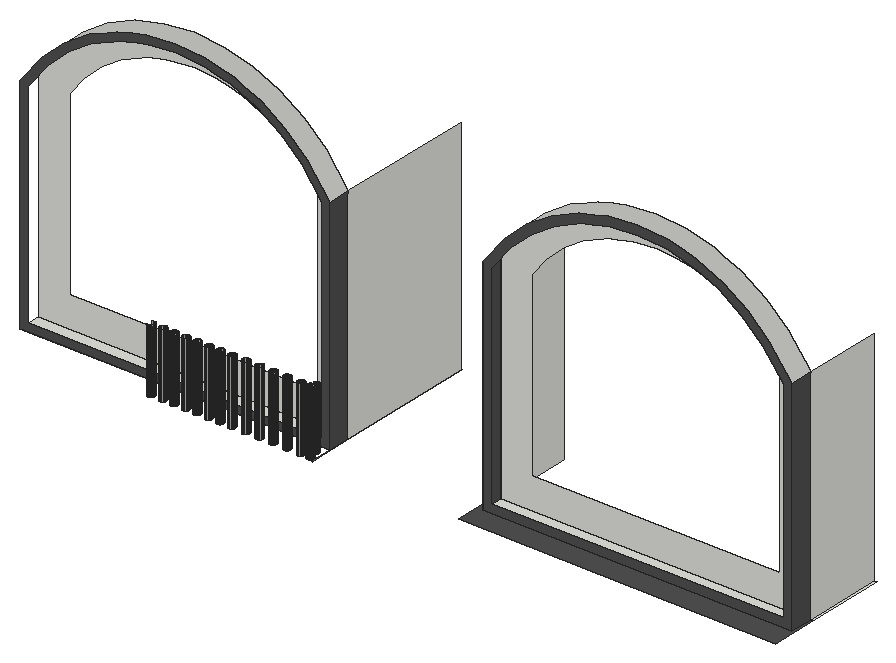
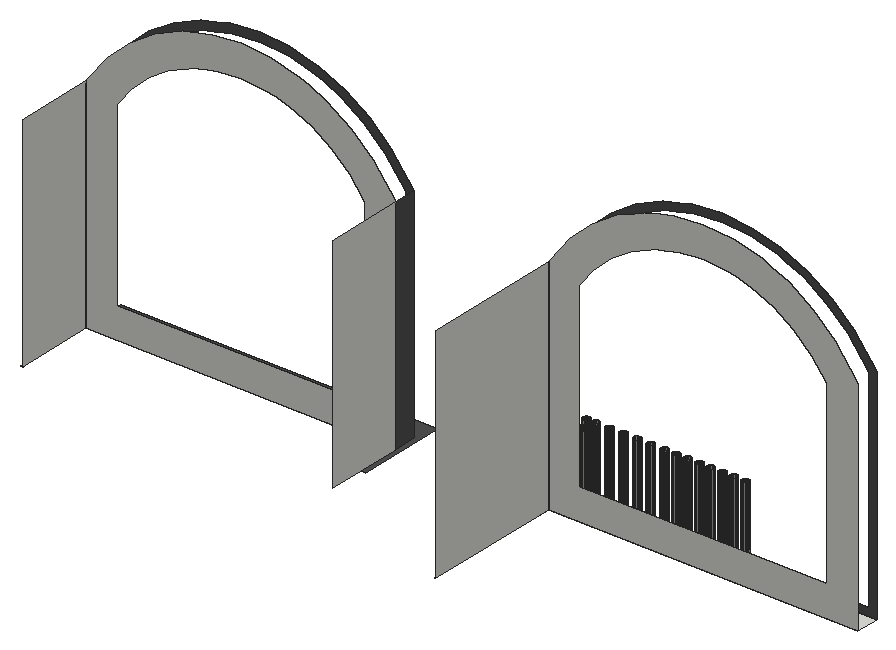
# SketchUp Ruby script. Lengths in inches.
U = 1.inch
M = Sketchup.active_model
def pt(a) = Geom::Point3d.new(a.map { |v| v * U })
def face(e, loops, mat)
  f = e.add_face(loops[0].map { |a| pt(a) })
  loops[1..].each { |l| e.add_face(l.map { |a| pt(a) }).erase! }
  f.material = f.back_material = mat if mat
  f
end
# faces: each face lists its corners as indices into pts; further lists are holes
def faces(e, pts, list, mat = nil) = list.each { |f| face(e, (f[0].is_a?(Array) ? f : [f]).map { |l| l.map { |i| pts[i] } }, mat) }
# xy, xz, yz: faces in a plane at the given z, y or x. An outline is a flat list of corners, or four numbers for a rectangle; further outlines are holes
def ring(l) = l.size == 4 ? [[l[0], l[1]], [l[2], l[1]], [l[2], l[3]], [l[0], l[3]]] : l.each_slice(2).to_a
def flat(e, list, mat, &to3) = list.each { |f| face(e, (f[0].is_a?(Array) ? f : [f]).map { |l| ring(l).map { |u, v| to3.(u, v) } }, mat) }
def xy(e, z, list, mat = nil) = flat(e, list, mat) { |x, y| [x, y, z] }
def xz(e, y, list, mat = nil) = flat(e, list, mat) { |x, z| [x, y, z] }
def yz(e, x, list, mat = nil) = flat(e, list, mat) { |y, z| [x, y, z] }
def lines(e, pts, list) = list.each { |a, b| e.add_line(pt(pts[a]), pt(pts[b])) }
# prism: a flat outline (further loops are holes) pulled along v
def prism(e, loops, v, mat = nil)
  f = face(e, loops, mat); d = Geom::Vector3d.new(v.map { |x| x * U })
  f.pushpull(f.normal.samedirection?(d) ? d.length : -d.length)
end
def box(e, o, s, mat = nil) = prism(e, [[o, [o[0] + s[0], o[1], o[2]], [o[0] + s[0], o[1] + s[1], o[2]], [o[0], o[1] + s[1], o[2]]]], [0, 0, s[2]], mat)
def at(x, y, z, deg = 0) = Geom::Transformation.translation(pt([x, y, z])) * Geom::Transformation.rotation(ORIGIN, Z_AXIS, deg.degrees)
def axes(o, x, y, z) = Geom::Transformation.new([*x, 0, *y, 0, *z, 0, *pt(o).to_a, 1])
def part(name) = M.definitions.add(name)
# library, detail: a bought-in or finely detailed component or shape, given as its bounding box
def library(name, o, s) = part(name).tap { |d| box(d.entities, o, s) }
def detail(e, o, s) = box(e.add_group.entities, o, s)
def put(e, d, t, mat = nil) = e.add_instance(d, t).tap { |i| i.material = mat if mat }
def group(e, t, mat = nil) = e.add_group.tap { |g| g.transformation = t; g.material = mat if mat }.entities
root = M.entities
M.materials.add("[0132_LightGray]").color = [169, 169, 169]
M.materials.add("[0135_DarkGray]").color = [81, 81, 81]
xy(root,638.72,[[299.83,31.93,299.47,31.97,299.14,32.11,298.86,32.33,298.64,32.62,298.5,32.95,298.45,33.3,298.5,33.66,298.64,33.99,298.86,34.28,299.14,34.49,299.47,34.63,299.83,34.68,300.18,34.63,300.52,34.49,300.8,34.28,301.02,33.99,301.16,33.66,301.2,33.3,301.16,32.95,301.02,32.62,300.8,32.33,300.52,32.11,300.18,31.97],[304.33,31.93,303.97,31.97,303.64,32.11,303.36,32.33,303.14,32.62,303,32.95,302.95,33.3,303,33.66,303.14,33.99,303.36,34.28,303.64,34.49,303.97,34.63,304.33,34.68,304.68,34.63,305.02,34.49,305.3,34.28,305.52,33.99,305.66,33.66,305.7,33.3,305.66,32.95,305.52,32.62,305.3,32.33,305.02,32.11,304.68,31.97],[308.83,31.93,308.47,31.97,308.14,32.11,307.86,32.33,307.64,32.62,307.5,32.95,307.45,33.3,307.5,33.66,307.64,33.99,307.86,34.28,308.14,34.49,308.47,34.63,308.83,34.68,309.18,34.63,309.52,34.49,309.8,34.28,310.02,33.99,310.16,33.66,310.2,33.3,310.16,32.95,310.02,32.62,309.8,32.33,309.52,32.11,309.18,31.97],[313.33,31.93,312.97,31.97,312.64,32.11,312.36,32.33,312.14,32.62,312,32.95,311.95,33.3,312,33.66,312.14,33.99,312.36,34.28,312.64,34.49,312.97,34.63,313.33,34.68,313.68,34.63,314.02,34.49,314.3,34.28,314.52,33.99,314.66,33.66,314.7,33.3,314.66,32.95,314.52,32.62,314.3,32.33,314.02,32.11,313.68,31.97],[317.83,31.93,317.47,31.97,317.14,32.11,316.86,32.33,316.64,32.62,316.5,32.95,316.45,33.3,316.5,33.66,316.64,33.99,316.86,34.28,317.14,34.49,317.47,34.63,317.83,34.68,318.18,34.63,318.52,34.49,318.8,34.28,319.02,33.99,319.16,33.66,319.2,33.3,319.16,32.95,319.02,32.62,318.8,32.33,318.52,32.11,318.18,31.97],
  [322.33,31.93,321.97,31.97,321.64,32.11,321.36,32.33,321.14,32.62,321,32.95,320.95,33.3,321,33.66,321.14,33.99,321.36,34.28,321.64,34.49,321.97,34.63,322.33,34.68,322.68,34.63,323.02,34.49,323.3,34.28,323.52,33.99,323.66,33.66,323.7,33.3,323.66,32.95,323.52,32.62,323.3,32.33,323.02,32.11,322.68,31.97],[326.83,31.93,326.47,31.97,326.14,32.11,325.86,32.33,325.64,32.62,325.5,32.95,325.45,33.3,325.5,33.66,325.64,33.99,325.86,34.28,326.14,34.49,326.47,34.63,326.83,34.68,327.18,34.63,327.52,34.49,327.8,34.28,328.02,33.99,328.16,33.66,328.2,33.3,328.16,32.95,328.02,32.62,327.8,32.33,327.52,32.11,327.18,31.97],[331.33,31.93,330.97,31.97,330.64,32.11,330.36,32.33,330.14,32.62,330,32.95,329.95,33.3,330,33.66,330.14,33.99,330.36,34.28,330.64,34.49,330.97,34.63,331.33,34.68,331.68,34.63,332.02,34.49,332.3,34.28,332.52,33.99,332.66,33.66,332.7,33.3,332.66,32.95,332.52,32.62,332.3,32.33,332.02,32.11,331.68,31.97],[336.7,31.93,336.35,31.97,336.02,32.11,335.73,32.33,335.51,32.62,335.375,32.95,335.33,33.3,335.375,33.66,335.51,33.99,335.73,34.28,336.02,34.49,336.35,34.63,336.7,34.68,337.06,34.63,337.39,34.49,337.68,34.28,337.89,33.99,338.03,33.66,338.08,33.3,338.03,32.95,337.89,32.62,337.68,32.33,337.39,32.11,337.06,31.97],[342.08,31.93,341.72,31.97,341.39,32.11,341.11,32.33,340.89,32.62,340.75,32.95,340.7,33.3,340.75,33.66,340.89,33.99,341.11,34.28,341.39,34.49,341.72,34.63,342.08,34.68,342.43,34.63,342.77,34.49,343.05,34.28,343.27,33.99,343.41,33.66,343.45,33.3,343.41,32.95,343.27,32.62,343.05,32.33,342.77,32.11,342.43,31.97],
  [347.45,31.93,347.1,31.97,346.77,32.11,346.48,32.33,346.26,32.62,346.125,32.95,346.08,33.3,346.125,33.66,346.26,33.99,346.48,34.28,346.77,34.49,347.1,34.63,347.45,34.68,347.81,34.63,348.14,34.49,348.43,34.28,348.64,33.99,348.78,33.66,348.83,33.3,348.78,32.95,348.64,32.62,348.43,32.33,348.14,32.11,347.81,31.97],[352.83,31.93,352.47,31.97,352.14,32.11,351.86,32.33,351.64,32.62,351.5,32.95,351.45,33.3,351.5,33.66,351.64,33.99,351.86,34.28,352.14,34.49,352.47,34.63,352.83,34.68,353.18,34.63,353.52,34.49,353.8,34.28,354.02,33.99,354.16,33.66,354.2,33.3,354.16,32.95,354.02,32.62,353.8,32.33,353.52,32.11,353.18,31.97],[358.2,31.93,357.85,31.97,357.52,32.11,357.23,32.33,357.01,32.62,356.875,32.95,356.83,33.3,356.875,33.66,357.01,33.99,357.23,34.28,357.52,34.49,357.85,34.63,358.2,34.68,358.56,34.63,358.89,34.49,359.18,34.28,359.39,33.99,359.53,33.66,359.58,33.3,359.53,32.95,359.39,32.62,359.18,32.33,358.89,32.11,358.56,31.97],[361.31,35.875,361.05,35.93,360.82,36.05,360.62,36.22,360.48,36.4375,360.4,36.6875,360.38,36.95,360.4375,37.2,360.55,37.4375,360.73,37.63,360.95,37.77,361.19,37.85,361.46,37.87,361.71,37.82,361.94,37.7,362.14,37.52,362.28,37.31,362.36,37.06,362.38,36.8,362.32,36.54,362.21,36.31,362.03,36.11,361.8125,35.97,361.57,35.89],[242.82,40.6875,363.51,49.6875],
  [423.07,40.6875,543.76,49.6875],[363.51,49.6875,363.89,104.375],[543.76,49.6875,543.95,80.4375],[543.95,49.6875,544.82,80.4375]])
xy(root,638.72,[[363.51,31.6875,363.89,37.6875],[421.14,31.6875,544.82,31.6875,544.82,49.6875,543.76,49.6875,543.76,40.6875,423.07,40.6875,423.07,66.75,421.14,66.75],[363.51,37.6875,363.89,49.6875]],"[0135_DarkGray]")
xz(root,40.6875,[[[242.82,638.72,363.51,638.72,363.51,725.13,354.58,736.74,346.11,744.61,336.46,750.96,329.5,754.04,325.89,755.63,320.02,757.13,314.6875,758.49,303.17,759.45,291.65,758.49,286.31,757.13,280.45,755.63,276.84,754.04,269.87,750.96,260.22,744.61,251.75,736.74,242.82,725.13],[245.76,641.66,245.76,724.14,253.93,734.75,262.04,742.29,271.28,748.38,278.02,751.35,281.41,752.85,287.03,754.28,292.13,755.58,303.17,756.5,314.2,755.58,319.3,754.28,324.92,752.85,328.3125,751.35,335.05,748.38,344.3,742.29,352.41,734.75,360.57,724.14,360.57,641.66]],[[423.07,638.72,543.76,638.72,543.76,725.13,534.83,736.74,526.36,744.61,516.71,750.96,509.75,754.04,506.14,755.63,500.27,757.13,494.9375,758.49,483.42,759.45,471.9,758.49,466.56,757.13,460.7,755.63,457.09,754.04,450.12,750.96,440.47,744.61,432,736.74,423.07,725.13],[426.42,642.07,426.42,724,434.48,734.47,442.54,741.96,451.73,748.01,458.4375,750.98,461.79,752.46,467.39,753.88,472.45,755.17,483.42,756.09,494.38,755.17,499.45,753.88,505.04,752.46,508.39,750.98,515.1,748.01,524.29,741.96,532.35,734.47,540.41,724,540.41,642.07]]],"[0135_DarkGray]")
xz(root,49.6875,[[[242.82,638.72,242.82,725.13,251.75,736.74,260.22,744.61,269.87,750.96,276.84,754.04,280.45,755.63,286.31,757.13,291.65,758.49,303.17,759.45,314.6875,758.49,320.02,757.13,325.89,755.63,329.5,754.04,336.46,750.96,346.11,744.61,354.58,736.74,363.51,725.13,363.51,638.72],[254.82,650.72,351.51,650.72,351.51,721.05,345.68,728.63,338.68,735.13,330.7,740.39,324.65,743.0625,321.95,744.25,317.06,745.5,312.69,746.61,311.64,746.7,305.64,747.2,303.17,747.41,293.64,746.61,289.27,745.5,284.38,744.25,281.68,743.0625,275.64,740.39,267.65,735.13,260.65,728.63,254.82,721.05]],[[423.07,638.72,423.07,725.13,432,736.74,440.47,744.61,450.12,750.96,457.09,754.04,460.7,755.63,466.56,757.13,471.9,758.49,483.42,759.45,494.9375,758.49,500.27,757.13,506.14,755.63,509.75,754.04,516.71,750.96,526.36,744.61,534.83,736.74,543.76,725.13,543.76,638.72],[435.07,650.72,531.76,650.72,531.76,721.05,525.93,728.63,518.93,735.13,510.95,740.39,504.9,743.0625,502.2,744.25,497.31,745.5,492.94,746.61,483.7,747.38,483.42,747.41,473.89,746.61,469.52,745.5,464.63,744.25,461.93,743.0625,455.89,740.39,447.9,735.13,440.9,728.63,435.07,721.05]]])
yz(root,363.51,[[49.6875,638.72,104.375,725.13]])
yz(root,363.51,[[40.6875,638.72,49.6875,725.13]],"[0135_DarkGray]")
yz(root,423.07,[[49.6875,638.72,80.4375,725.13]])
yz(root,423.07,[[40.6875,638.72,49.6875,725.13]],"[0135_DarkGray]")
yz(root,543.76,[[49.6875,638.72,80.4375,725.13]])
yz(root,543.76,[[40.6875,638.72,49.6875,725.13]],"[0135_DarkGray]")
p = [[299.47,31.97,638.72],[299.83,31.93,638.72],[299.83,31.93,663.85],[299.47,31.97,663.85],[300.18,31.97,638.72],[300.18,31.97,663.85],
  [303.97,31.97,638.72],[304.33,31.93,638.72],[304.33,31.93,663.85],[303.97,31.97,663.85],[304.68,31.97,638.72],[304.68,31.97,663.85],
  [308.47,31.97,638.72],[308.83,31.93,638.72],[308.83,31.93,663.85],[308.47,31.97,663.85],[309.18,31.97,638.72],[309.18,31.97,663.85],
  [312.97,31.97,638.72],[313.33,31.93,638.72],[313.33,31.93,663.85],[312.97,31.97,663.85],[313.68,31.97,638.72],[313.68,31.97,663.85],
  [317.47,31.97,638.72],[317.83,31.93,638.72],[317.83,31.93,663.85],[317.47,31.97,663.85],[318.18,31.97,638.72],[318.18,31.97,663.85],
  [321.97,31.97,638.72],[322.33,31.93,638.72],[322.33,31.93,663.85],[321.97,31.97,663.85],[322.68,31.97,638.72],[322.68,31.97,663.85],
  [326.47,31.97,638.72],[326.83,31.93,638.72],[326.83,31.93,663.85],[326.47,31.97,663.85],[327.18,31.97,638.72],[327.18,31.97,663.85],
  [330.97,31.97,638.72],[331.33,31.93,638.72],[331.33,31.93,663.85],[330.97,31.97,663.85],[331.68,31.97,638.72],[331.68,31.97,663.85],
  [336.35,31.97,638.72],[336.7,31.93,638.72],[336.7,31.93,663.85],[336.35,31.97,663.85],[337.06,31.97,638.72],[337.06,31.97,663.85],
  [341.72,31.97,638.72],[342.08,31.93,638.72],[342.08,31.93,663.85],[341.72,31.97,663.85],[342.43,31.97,638.72],[342.43,31.97,663.85],
  [347.1,31.97,638.72],[347.45,31.93,638.72],[347.45,31.93,663.85],[347.1,31.97,663.85],[347.81,31.97,638.72],[347.81,31.97,663.85],
  [352.47,31.97,638.72],[352.83,31.93,638.72],[352.83,31.93,663.85],[352.47,31.97,663.85],[353.18,31.97,638.72],[353.18,31.97,663.85],
  [357.85,31.97,638.72],[358.2,31.93,638.72],[358.2,31.93,663.85],[357.85,31.97,663.85],[358.56,31.97,638.72],[358.56,31.97,663.85],
  [361.53,31.97,638.72],[361.89,31.93,638.72],[361.89,31.93,663.85],[361.53,31.97,663.85],[362.25,31.97,638.72],[362.25,31.97,663.85],
  [299.14,32.11,638.72],[299.14,32.11,663.85],[300.52,32.11,638.72],[300.52,32.11,663.85],[303.64,32.11,638.72],[303.64,32.11,663.85],
  [305.02,32.11,638.72],[305.02,32.11,663.85],[308.14,32.11,638.72],[308.14,32.11,663.85],[309.52,32.11,638.72],[309.52,32.11,663.85],
  [312.64,32.11,638.72],[312.64,32.11,663.85],[314.02,32.11,638.72],[314.02,32.11,663.85],[317.14,32.11,638.72],[317.14,32.11,663.85],
  [318.52,32.11,638.72],[318.52,32.11,663.85],[321.64,32.11,638.72],[321.64,32.11,663.85],[323.02,32.11,638.72],[323.02,32.11,663.85],
  [326.14,32.11,638.72],[326.14,32.11,663.85],[327.52,32.11,638.72],[327.52,32.11,663.85],[330.64,32.11,638.72],[330.64,32.11,663.85],
  [332.02,32.11,638.72],[332.02,32.11,663.85],[336.02,32.11,638.72],[336.02,32.11,663.85],[337.39,32.11,638.72],[337.39,32.11,663.85],
  [341.39,32.11,638.72],[341.39,32.11,663.85],[342.77,32.11,638.72],[342.77,32.11,663.85],[346.77,32.11,638.72],[346.77,32.11,663.85],
  [348.14,32.11,638.72],[348.14,32.11,663.85],[352.14,32.11,638.72],[352.14,32.11,663.85],[353.52,32.11,638.72],[353.52,32.11,663.85],
  [357.52,32.11,638.72],[357.52,32.11,663.85],[358.89,32.11,638.72],[358.89,32.11,663.85],[361.2,32.11,638.72],[361.2,32.11,663.85],
  [362.58,32.11,638.72],[362.58,32.11,663.85],[300.8,32.33,638.72],[300.8,32.33,663.85],[303.36,32.33,638.72],[303.36,32.33,663.85],
  [305.3,32.33,638.72],[305.3,32.33,663.85],[307.86,32.33,638.72],[307.86,32.33,663.85],[309.8,32.33,638.72],[309.8,32.33,663.85],
  [312.36,32.33,638.72],[312.36,32.33,663.85],[314.3,32.33,638.72],[314.3,32.33,663.85],[316.86,32.33,638.72],[316.86,32.33,663.85],
  [318.8,32.33,638.72],[318.8,32.33,663.85],[321.36,32.33,638.72],[321.36,32.33,663.85],[323.3,32.33,638.72],[323.3,32.33,663.85],
  [325.86,32.33,638.72],[325.86,32.33,663.85],[327.8,32.33,638.72],[327.8,32.33,663.85],[330.36,32.33,638.72],[330.36,32.33,663.85],
  [332.3,32.33,638.72],[332.3,32.33,663.85],[335.73,32.33,638.72],[335.73,32.33,663.85],[337.68,32.33,638.72],[337.68,32.33,663.85],
  [341.11,32.33,638.72],[341.11,32.33,663.85],[343.05,32.33,638.72],[343.05,32.33,663.85],[346.48,32.33,638.72],[346.48,32.33,663.85],
  [348.43,32.33,638.72],[348.43,32.33,663.85],[351.86,32.33,638.72],[351.86,32.33,663.85],[353.8,32.33,638.72],[353.8,32.33,663.85],
  [357.23,32.33,638.72],[357.23,32.33,663.85],[359.18,32.33,638.72],[359.18,32.33,663.85],[360.92,32.33,638.72],[360.92,32.33,663.85],
  [362.86,32.33,638.72],[362.86,32.33,663.85],[301.02,32.62,638.72],[301.02,32.62,663.85],[303.14,32.62,638.72],[303.14,32.62,663.85],
  [305.52,32.62,638.72],[305.52,32.62,663.85],[307.64,32.62,638.72],[307.64,32.62,663.85],[310.02,32.62,638.72],[310.02,32.62,663.85],
  [312.14,32.62,638.72],[312.14,32.62,663.85],[314.52,32.62,638.72],[314.52,32.62,663.85],[316.64,32.62,638.72],[316.64,32.62,663.85],
  [319.02,32.62,638.72],[319.02,32.62,663.85],[321.14,32.62,638.72],[321.14,32.62,663.85],[323.52,32.62,638.72],[323.52,32.62,663.85],
  [325.64,32.62,638.72],[325.64,32.62,663.85],[328.02,32.62,638.72],[328.02,32.62,663.85],[330.14,32.62,638.72],[330.14,32.62,663.85],
  [332.52,32.62,638.72],[332.52,32.62,663.85],[335.51,32.62,638.72],[335.51,32.62,663.85],[337.89,32.62,638.72],[337.89,32.62,663.85],
  [340.89,32.62,638.72],[340.89,32.62,663.85],[343.27,32.62,638.72],[343.27,32.62,663.85],[346.26,32.62,638.72],[346.26,32.62,663.85],
  [348.64,32.62,638.72],[348.64,32.62,663.85],[351.64,32.62,638.72],[351.64,32.62,663.85],[354.02,32.62,638.72],[354.02,32.62,663.85],
  [357.01,32.62,638.72],[357.01,32.62,663.85],[359.39,32.62,638.72],[359.39,32.62,663.85],[360.7,32.62,638.72],[360.7,32.62,663.85],
  [363.08,32.62,638.72],[363.08,32.62,663.85],[301.16,32.95,638.72],[301.16,32.95,663.85],[303,32.95,638.72],[303,32.95,663.85],
  [305.66,32.95,638.72],[305.66,32.95,663.85],[307.5,32.95,638.72],[307.5,32.95,663.85],[310.16,32.95,638.72],[310.16,32.95,663.85],
  [312,32.95,638.72],[312,32.95,663.85],[314.66,32.95,638.72],[314.66,32.95,663.85],[316.5,32.95,638.72],[316.5,32.95,663.85],
  [319.16,32.95,638.72],[319.16,32.95,663.85],[321,32.95,638.72],[321,32.95,663.85],[323.66,32.95,638.72],[323.66,32.95,663.85],
  [325.5,32.95,638.72],[325.5,32.95,663.85],[328.16,32.95,638.72],[328.16,32.95,663.85],[330,32.95,638.72],[330,32.95,663.85],
  [332.66,32.95,638.72],[332.66,32.95,663.85],[335.375,32.95,638.72],[335.375,32.95,663.85],[338.03,32.95,638.72],[338.03,32.95,663.85],
  [340.75,32.95,638.72],[340.75,32.95,663.85],[343.41,32.95,638.72],[343.41,32.95,663.85],[346.125,32.95,638.72],[346.125,32.95,663.85],
  [348.78,32.95,638.72],[348.78,32.95,663.85],[351.5,32.95,638.72],[351.5,32.95,663.85],[354.16,32.95,638.72],[354.16,32.95,663.85],
  [356.875,32.95,638.72],[356.875,32.95,663.85],[359.53,32.95,638.72],[359.53,32.95,663.85],[360.5625,32.95,638.72],[360.5625,32.95,663.85],
  [363.22,32.95,638.72],[363.22,32.95,663.85],[301.2,33.3,638.72],[301.2,33.3,663.85],[302.95,33.3,638.72],[302.95,33.3,663.85],
  [305.7,33.3,638.72],[305.7,33.3,663.85],[307.45,33.3,638.72],[307.45,33.3,663.85],[310.2,33.3,638.72],[310.2,33.3,663.85],
  [311.95,33.3,638.72],[311.95,33.3,663.85],[314.7,33.3,638.72],[314.7,33.3,663.85],[316.45,33.3,638.72],[316.45,33.3,663.85],
  [319.2,33.3,638.72],[319.2,33.3,663.85],[320.95,33.3,638.72],[320.95,33.3,663.85],[323.7,33.3,638.72],[323.7,33.3,663.85],
  [325.45,33.3,638.72],[325.45,33.3,663.85],[328.2,33.3,638.72],[328.2,33.3,663.85],[329.95,33.3,638.72],[329.95,33.3,663.85],
  [332.7,33.3,638.72],[332.7,33.3,663.85],[335.33,33.3,638.72],[335.33,33.3,663.85],[338.08,33.3,638.72],[338.08,33.3,663.85],
  [340.7,33.3,638.72],[340.7,33.3,663.85],[343.45,33.3,638.72],[343.45,33.3,663.85],[346.08,33.3,638.72],[346.08,33.3,663.85],
  [348.83,33.3,638.72],[348.83,33.3,663.85],[351.45,33.3,638.72],[351.45,33.3,663.85],[354.2,33.3,638.72],[354.2,33.3,663.85],
  [356.83,33.3,638.72],[356.83,33.3,663.85],[359.58,33.3,638.72],[359.58,33.3,663.85],[360.52,33.3,638.72],[360.52,33.3,663.85],
  [363.27,33.3,638.72],[363.27,33.3,663.85],[301.16,33.66,638.72],[301.16,33.66,663.85],[303,33.66,638.72],[303,33.66,663.85],
  [305.66,33.66,638.72],[305.66,33.66,663.85],[307.5,33.66,638.72],[307.5,33.66,663.85],[310.16,33.66,638.72],[310.16,33.66,663.85],
  [312,33.66,638.72],[312,33.66,663.85],[314.66,33.66,638.72],[314.66,33.66,663.85],[316.5,33.66,638.72],[316.5,33.66,663.85],
  [319.16,33.66,638.72],[319.16,33.66,663.85],[321,33.66,638.72],[321,33.66,663.85],[323.66,33.66,638.72],[323.66,33.66,663.85],
  [325.5,33.66,638.72],[325.5,33.66,663.85],[328.16,33.66,638.72],[328.16,33.66,663.85],[330,33.66,638.72],[330,33.66,663.85],
  [332.66,33.66,638.72],[332.66,33.66,663.85],[335.375,33.66,638.72],[335.375,33.66,663.85],[338.03,33.66,638.72],[338.03,33.66,663.85],
  [340.75,33.66,638.72],[340.75,33.66,663.85],[343.41,33.66,638.72],[343.41,33.66,663.85],[346.125,33.66,638.72],[346.125,33.66,663.85],
  [348.78,33.66,638.72],[348.78,33.66,663.85],[351.5,33.66,638.72],[351.5,33.66,663.85],[354.16,33.66,638.72],[354.16,33.66,663.85],
  [356.875,33.66,638.72],[356.875,33.66,663.85],[359.53,33.66,638.72],[359.53,33.66,663.85],[360.5625,33.66,638.72],[360.5625,33.66,663.85],
  [363.22,33.66,638.72],[363.22,33.66,663.85],[301.02,33.99,638.72],[301.02,33.99,663.85],[303.14,33.99,638.72],[303.14,33.99,663.85],
  [305.52,33.99,638.72],[305.52,33.99,663.85],[307.64,33.99,638.72],[307.64,33.99,663.85],[310.02,33.99,638.72],[310.02,33.99,663.85],
  [312.14,33.99,638.72],[312.14,33.99,663.85],[314.52,33.99,638.72],[314.52,33.99,663.85],[316.64,33.99,638.72],[316.64,33.99,663.85],
  [319.02,33.99,638.72],[319.02,33.99,663.85],[321.14,33.99,638.72],[321.14,33.99,663.85],[323.52,33.99,638.72],[323.52,33.99,663.85],
  [325.64,33.99,638.72],[325.64,33.99,663.85],[328.02,33.99,638.72],[328.02,33.99,663.85],[330.14,33.99,638.72],[330.14,33.99,663.85],
  [332.52,33.99,638.72],[332.52,33.99,663.85],[335.51,33.99,638.72],[335.51,33.99,663.85],[337.89,33.99,638.72],[337.89,33.99,663.85],
  [340.89,33.99,638.72],[340.89,33.99,663.85],[343.27,33.99,638.72],[343.27,33.99,663.85],[346.26,33.99,638.72],[346.26,33.99,663.85],
  [348.64,33.99,638.72],[348.64,33.99,663.85],[351.64,33.99,638.72],[351.64,33.99,663.85],[354.02,33.99,638.72],[354.02,33.99,663.85],
  [357.01,33.99,638.72],[357.01,33.99,663.85],[359.39,33.99,638.72],[359.39,33.99,663.85],[360.7,33.99,638.72],[360.7,33.99,663.85],
  [363.08,33.99,638.72],[363.08,33.99,663.85],[300.8,34.28,638.72],[300.8,34.28,663.85],[303.36,34.28,638.72],[303.36,34.28,663.85],
  [305.3,34.28,638.72],[305.3,34.28,663.85],[307.86,34.28,638.72],[307.86,34.28,663.85],[309.8,34.28,638.72],[309.8,34.28,663.85],
  [312.36,34.28,638.72],[312.36,34.28,663.85],[314.3,34.28,638.72],[314.3,34.28,663.85],[316.86,34.28,638.72],[316.86,34.28,663.85],
  [318.8,34.28,638.72],[318.8,34.28,663.85],[321.36,34.28,638.72],[321.36,34.28,663.85],[323.3,34.28,638.72],[323.3,34.28,663.85],
  [325.86,34.28,638.72],[325.86,34.28,663.85],[327.8,34.28,638.72],[327.8,34.28,663.85],[330.36,34.28,638.72],[330.36,34.28,663.85],
  [332.3,34.28,638.72],[332.3,34.28,663.85],[335.73,34.28,638.72],[335.73,34.28,663.85],[337.68,34.28,638.72],[337.68,34.28,663.85],
  [341.11,34.28,638.72],[341.11,34.28,663.85],[343.05,34.28,638.72],[343.05,34.28,663.85],[346.48,34.28,638.72],[346.48,34.28,663.85],
  [348.43,34.28,638.72],[348.43,34.28,663.85],[351.86,34.28,638.72],[351.86,34.28,663.85],[353.8,34.28,638.72],[353.8,34.28,663.85],
  [357.23,34.28,638.72],[357.23,34.28,663.85],[359.18,34.28,638.72],[359.18,34.28,663.85],[360.92,34.28,638.72],[360.92,34.28,663.85],
  [362.86,34.28,638.72],[362.86,34.28,663.85],[300.52,34.49,638.72],[300.52,34.49,663.85],[303.64,34.49,638.72],[303.64,34.49,663.85],
  [305.02,34.49,638.72],[305.02,34.49,663.85],[308.14,34.49,638.72],[308.14,34.49,663.85],[309.52,34.49,638.72],[309.52,34.49,663.85],
  [312.64,34.49,638.72],[312.64,34.49,663.85],[314.02,34.49,638.72],[314.02,34.49,663.85],[317.14,34.49,638.72],[317.14,34.49,663.85],
  [318.52,34.49,638.72],[318.52,34.49,663.85],[321.64,34.49,638.72],[321.64,34.49,663.85],[323.02,34.49,638.72],[323.02,34.49,663.85],
  [326.14,34.49,638.72],[326.14,34.49,663.85],[327.52,34.49,638.72],[327.52,34.49,663.85],[330.64,34.49,638.72],[330.64,34.49,663.85],
  [332.02,34.49,638.72],[332.02,34.49,663.85],[336.02,34.49,638.72],[336.02,34.49,663.85],[337.39,34.49,638.72],[337.39,34.49,663.85],
  [341.39,34.49,638.72],[341.39,34.49,663.85],[342.77,34.49,638.72],[342.77,34.49,663.85],[346.77,34.49,638.72],[346.77,34.49,663.85],
  [348.14,34.49,638.72],[348.14,34.49,663.85],[352.14,34.49,638.72],[352.14,34.49,663.85],[353.52,34.49,638.72],[353.52,34.49,663.85],
  [357.52,34.49,638.72],[357.52,34.49,663.85],[358.89,34.49,638.72],[358.89,34.49,663.85],[361.2,34.49,638.72],[361.2,34.49,663.85],
  [362.58,34.49,638.72],[362.58,34.49,663.85],[299.47,34.63,638.72],[299.14,34.49,638.72],[299.14,34.49,663.85],[299.47,34.63,663.85],
  [300.18,34.63,638.72],[300.18,34.63,663.85],[303.97,34.63,638.72],[303.97,34.63,663.85],[304.68,34.63,638.72],[304.68,34.63,663.85],
  [308.47,34.63,638.72],[308.47,34.63,663.85],[309.18,34.63,638.72],[309.18,34.63,663.85],[312.97,34.63,638.72],[312.97,34.63,663.85],
  [313.68,34.63,638.72],[313.68,34.63,663.85],[317.47,34.63,638.72],[317.47,34.63,663.85],[318.18,34.63,638.72],[318.18,34.63,663.85],
  [321.97,34.63,638.72],[321.97,34.63,663.85],[322.68,34.63,638.72],[322.68,34.63,663.85],[326.47,34.63,638.72],[326.47,34.63,663.85],
  [327.18,34.63,638.72],[327.18,34.63,663.85],[330.97,34.63,638.72],[330.97,34.63,663.85],[331.68,34.63,638.72],[331.68,34.63,663.85],
  [336.35,34.63,638.72],[336.35,34.63,663.85],[337.06,34.63,638.72],[337.06,34.63,663.85],[341.72,34.63,638.72],[341.72,34.63,663.85],
  [342.43,34.63,638.72],[342.43,34.63,663.85],[347.1,34.63,638.72],[347.1,34.63,663.85],[347.81,34.63,638.72],[347.81,34.63,663.85],
  [352.47,34.63,638.72],[352.47,34.63,663.85],[353.18,34.63,638.72],[353.18,34.63,663.85],[357.85,34.63,638.72],[357.85,34.63,663.85],
  [358.56,34.63,638.72],[358.56,34.63,663.85],[361.53,34.63,638.72],[361.53,34.63,663.85],[362.25,34.63,638.72],[362.25,34.63,663.85],
  [299.83,34.68,638.72],[299.83,34.68,663.85],[304.33,34.68,638.72],[304.33,34.68,663.85],[308.83,34.68,638.72],[308.83,34.68,663.85],
  [313.33,34.68,638.72],[313.33,34.68,663.85],[317.83,34.68,638.72],[317.83,34.68,663.85],[322.33,34.68,638.72],[322.33,34.68,663.85],
  [326.83,34.68,638.72],[326.83,34.68,663.85],[331.33,34.68,638.72],[331.33,34.68,663.85],[336.7,34.68,638.72],[336.7,34.68,663.85],
  [342.08,34.68,638.72],[342.08,34.68,663.85],[347.45,34.68,638.72],[347.45,34.68,663.85],[352.83,34.68,638.72],[352.83,34.68,663.85],
  [358.2,34.68,638.72],[358.2,34.68,663.85],[361.89,34.68,638.72],[361.89,34.68,663.85],[360.82,36.05,638.72],[361.05,35.93,638.72],
  [361.05,35.93,662.87],[360.82,36.05,662.87],[361.31,35.875,638.72],[361.31,35.875,662.87],[361.57,35.89,638.72],[361.57,35.89,662.87],
  [361.8125,35.97,638.72],[361.8125,35.97,662.87],[360.62,36.22,638.72],[360.62,36.22,662.87],[362.03,36.11,638.72],[362.03,36.11,662.87],
  [362.21,36.31,638.72],[362.21,36.31,662.87],[360.48,36.4375,638.72],[360.48,36.4375,662.87],[362.32,36.54,638.72],[362.32,36.54,662.87],
  [360.4,36.6875,638.72],[360.4,36.6875,662.87],[362.38,36.8,638.72],[362.38,36.8,662.87],[360.38,36.95,638.72],[360.38,36.95,662.87],
  [362.36,37.06,638.72],[362.36,37.06,662.87],[360.4375,37.2,638.72],[360.4375,37.2,662.87],[362.28,37.31,638.72],[362.28,37.31,662.87],
  [360.55,37.4375,638.72],[360.55,37.4375,662.87],[362.14,37.52,638.72],[362.14,37.52,662.87],[360.73,37.63,638.72],[360.73,37.63,662.87],
  [361.94,37.7,638.72],[361.94,37.7,662.87],[360.95,37.77,638.72],[360.95,37.77,662.87],[361.71,37.82,638.72],[361.71,37.82,662.87],
  [361.19,37.85,638.72],[361.19,37.85,662.87],[361.46,37.87,638.72],[361.46,37.87,662.87]]
faces(root,p,[[0,1,2,3],[1,4,5,2],[6,7,8,9],[7,10,11,8],[12,13,14,15],[13,16,17,14],[18,19,20,21],[19,22,23,20],
  [24,25,26,27],[25,28,29,26],[30,31,32,33],[31,34,35,32],[36,37,38,39],[37,40,41,38],[42,43,44,45],[43,46,47,44],
  [48,49,50,51],[49,52,53,50],[54,55,56,57],[55,58,59,56],[60,61,62,63],[61,64,65,62],[66,67,68,69],[67,70,71,68],
  [72,73,74,75],[73,76,77,74],[78,79,80,81],[79,82,83,80],[84,0,3,85],[4,86,87,5],[88,6,9,89],[10,90,91,11],
  [92,12,15,93],[16,94,95,17],[96,18,21,97],[22,98,99,23],[100,24,27,101],[28,102,103,29],[104,30,33,105],[34,106,107,35],
  [108,36,39,109],[40,110,111,41],[112,42,45,113],[46,114,115,47],[116,48,51,117],[52,118,119,53],[120,54,57,121],[58,122,123,59],
  [124,60,63,125],[64,126,127,65],[128,66,69,129],[70,130,131,71],[132,72,75,133],[76,134,135,77],[136,78,81,137],[82,138,139,83],
  [86,140,141,87],[142,88,89,143],[90,144,145,91],[146,92,93,147],[94,148,149,95],[150,96,97,151],[98,152,153,99],[154,100,101,155],
  [102,156,157,103],[158,104,105,159],[106,160,161,107],[162,108,109,163],[110,164,165,111],[166,112,113,167],[114,168,169,115],[170,116,117,171],
  [118,172,173,119],[174,120,121,175],[122,176,177,123],[178,124,125,179],[126,180,181,127],[182,128,129,183],[130,184,185,131],[186,132,133,187],
  [134,188,189,135],[190,136,137,191],[138,192,193,139],[140,194,195,141],[196,142,143,197],[144,198,199,145],[200,146,147,201],[148,202,203,149],
  [204,150,151,205],[152,206,207,153],[208,154,155,209],[156,210,211,157],[212,158,159,213],[160,214,215,161],[216,162,163,217],[164,218,219,165],
  [220,166,167,221],[168,222,223,169],[224,170,171,225],[172,226,227,173],[228,174,175,229],[176,230,231,177],[232,178,179,233],[180,234,235,181],
  [236,182,183,237],[184,238,239,185],[240,186,187,241],[188,242,243,189],[244,190,191,245],[192,246,247,193],[194,248,249,195],[250,196,197,251],
  [198,252,253,199],[254,200,201,255],[202,256,257,203],[258,204,205,259],[206,260,261,207],[262,208,209,263],[210,264,265,211],[266,212,213,267],
  [214,268,269,215],[270,216,217,271],[218,272,273,219],[274,220,221,275],[222,276,277,223],[278,224,225,279],[226,280,281,227],[282,228,229,283],
  [230,284,285,231],[286,232,233,287],[234,288,289,235],[290,236,237,291],[238,292,293,239],[294,240,241,295],[242,296,297,243],[298,244,245,299],
  [246,300,301,247],[248,302,303,249],[304,250,251,305],[252,306,307,253],[308,254,255,309],[256,310,311,257],[312,258,259,313],[260,314,315,261],
  [316,262,263,317],[264,318,319,265],[320,266,267,321],[268,322,323,269],[324,270,271,325],[272,326,327,273],[328,274,275,329],[276,330,331,277],
  [332,278,279,333],[280,334,335,281],[336,282,283,337],[284,338,339,285],[340,286,287,341],[288,342,343,289],[344,290,291,345],[292,346,347,293],
  [348,294,295,349],[296,350,351,297],[352,298,299,353],[300,354,355,301],[302,356,357,303],[358,304,305,359],[306,360,361,307],[362,308,309,363],
  [310,364,365,311],[366,312,313,367],[314,368,369,315],[370,316,317,371],[318,372,373,319],[374,320,321,375],[322,376,377,323],[378,324,325,379],
  [326,380,381,327],[382,328,329,383],[330,384,385,331],[386,332,333,387],[334,388,389,335],[390,336,337,391],[338,392,393,339],[394,340,341,395],
  [342,396,397,343],[398,344,345,399],[346,400,401,347],[402,348,349,403],[350,404,405,351],[406,352,353,407],[354,408,409,355],[356,410,411,357],
  [412,358,359,413],[360,414,415,361],[416,362,363,417],[364,418,419,365],[420,366,367,421],[368,422,423,369],[424,370,371,425],[372,426,427,373],
  [428,374,375,429],[376,430,431,377],[432,378,379,433],[380,434,435,381],[436,382,383,437],[384,438,439,385],[440,386,387,441],[388,442,443,389],
  [444,390,391,445],[392,446,447,393],[448,394,395,449],[396,450,451,397],[452,398,399,453],[400,454,455,401],[456,402,403,457],[404,458,459,405],
  [460,406,407,461],[408,462,463,409],[410,464,465,411],[466,412,413,467],[414,468,469,415],[470,416,417,471],[418,472,473,419],[474,420,421,475],
  [422,476,477,423],[478,424,425,479],[426,480,481,427],[482,428,429,483],[430,484,485,431],[486,432,433,487],[434,488,489,435],[490,436,437,491],
  [438,492,493,439],[494,440,441,495],[442,496,497,443],[498,444,445,499],[446,500,501,447],[502,448,449,503],[450,504,505,451],[506,452,453,507],
  [454,508,509,455],[510,456,457,511],[458,512,513,459],[514,460,461,515],[462,516,517,463],[464,518,519,465],[520,466,467,521],[468,522,523,469],
  [524,470,471,525],[472,526,527,473],[528,474,475,529],[476,530,531,477],[532,478,479,533],[480,534,535,481],[536,482,483,537],[484,538,539,485],
  [540,486,487,541],[488,542,543,489],[544,490,491,545],[492,546,547,493],[548,494,495,549],[496,550,551,497],[552,498,499,553],[500,554,555,501],
  [556,502,503,557],[504,558,559,505],[560,506,507,561],[508,562,563,509],[564,510,511,565],[512,566,567,513],[568,514,515,569],[516,570,571,517],
  [572,573,574,575],[518,576,577,519],[578,520,521,579],[522,580,581,523],[582,524,525,583],[526,584,585,527],[586,528,529,587],[530,588,589,531],
  [590,532,533,591],[534,592,593,535],[594,536,537,595],[538,596,597,539],[598,540,541,599],[542,600,601,543],[602,544,545,603],[546,604,605,547],
  [606,548,549,607],[550,608,609,551],[610,552,553,611],[554,612,613,555],[614,556,557,615],[558,616,617,559],[618,560,561,619],[562,620,621,563],
  [622,564,565,623],[566,624,625,567],[626,568,569,627],[570,628,629,571],[630,572,575,631],[576,630,631,577],[632,578,579,633],[580,632,633,581],
  [634,582,583,635],[584,634,635,585],[636,586,587,637],[588,636,637,589],[638,590,591,639],[592,638,639,593],[640,594,595,641],[596,640,641,597],
  [642,598,599,643],[600,642,643,601],[644,602,603,645],[604,644,645,605],[646,606,607,647],[608,646,647,609],[648,610,611,649],[612,648,649,613],
  [650,614,615,651],[616,650,651,617],[652,618,619,653],[620,652,653,621],[654,622,623,655],[624,654,655,625],[656,626,627,657],[628,656,657,629],
  [658,659,660,661],[659,662,663,660],[662,664,665,663],[664,666,667,665],[668,658,661,669],[666,670,671,667],[670,672,673,671],[674,668,669,675],
  [672,676,677,673],[678,674,675,679],[676,680,681,677],[682,678,679,683],[680,684,685,681],[686,682,683,687],[684,688,689,685],[690,686,687,691],
  [688,692,693,689],[694,690,691,695],[692,696,697,693],[698,694,695,699],[696,700,701,697],[702,698,699,703],[700,704,705,701],[704,702,703,705]],"[0132_LightGray]")
